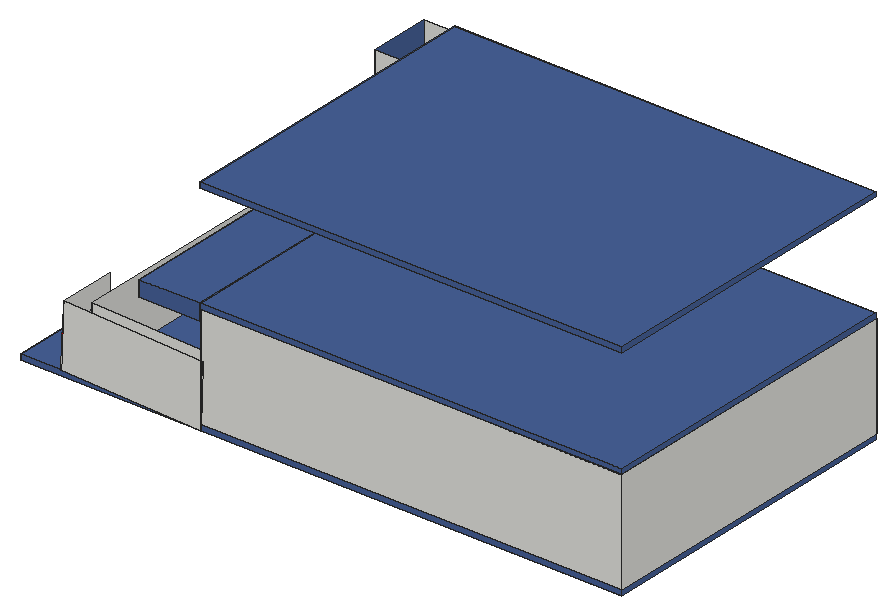
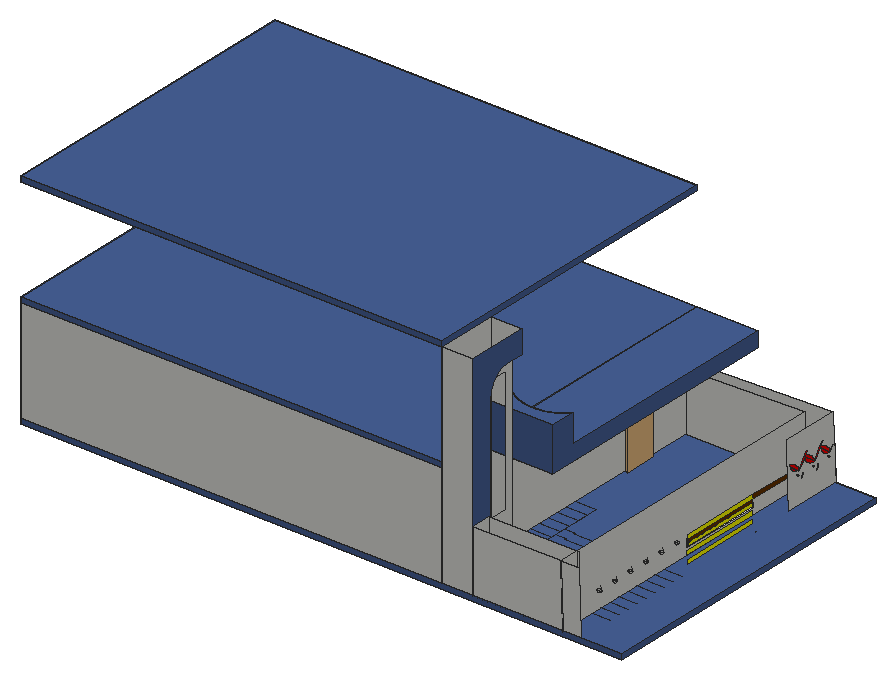
# SketchUp Ruby script. Lengths in inches.
U = 1.inch
M = Sketchup.active_model
def pt(a) = Geom::Point3d.new(a.map { |v| v * U })
def face(e, loops, mat)
  f = e.add_face(loops[0].map { |a| pt(a) })
  loops[1..].each { |l| e.add_face(l.map { |a| pt(a) }).erase! }
  f.material = f.back_material = mat if mat
  f
end
# faces: each face lists its corners as indices into pts; further lists are holes
def faces(e, pts, list, mat = nil) = list.each { |f| face(e, (f[0].is_a?(Array) ? f : [f]).map { |l| l.map { |i| pts[i] } }, mat) }
# xy, xz, yz: faces in a plane at the given z, y or x. An outline is a flat list of corners, or four numbers for a rectangle; further outlines are holes
def ring(l) = l.size == 4 ? [[l[0], l[1]], [l[2], l[1]], [l[2], l[3]], [l[0], l[3]]] : l.each_slice(2).to_a
def flat(e, list, mat, &to3) = list.each { |f| face(e, (f[0].is_a?(Array) ? f : [f]).map { |l| ring(l).map { |u, v| to3.(u, v) } }, mat) }
def xy(e, z, list, mat = nil) = flat(e, list, mat) { |x, y| [x, y, z] }
def xz(e, y, list, mat = nil) = flat(e, list, mat) { |x, z| [x, y, z] }
def yz(e, x, list, mat = nil) = flat(e, list, mat) { |y, z| [x, y, z] }
def lines(e, pts, list) = list.each { |a, b| e.add_line(pt(pts[a]), pt(pts[b])) }
# prism: a flat outline (further loops are holes) pulled along v
def prism(e, loops, v, mat = nil)
  f = face(e, loops, mat); d = Geom::Vector3d.new(v.map { |x| x * U })
  f.pushpull(f.normal.samedirection?(d) ? d.length : -d.length)
end
def box(e, o, s, mat = nil) = prism(e, [[o, [o[0] + s[0], o[1], o[2]], [o[0] + s[0], o[1] + s[1], o[2]], [o[0], o[1] + s[1], o[2]]]], [0, 0, s[2]], mat)
def at(x, y, z, deg = 0) = Geom::Transformation.translation(pt([x, y, z])) * Geom::Transformation.rotation(ORIGIN, Z_AXIS, deg.degrees)
def axes(o, x, y, z) = Geom::Transformation.new([*x, 0, *y, 0, *z, 0, *pt(o).to_a, 1])
def part(name) = M.definitions.add(name)
# library, detail: a bought-in or finely detailed component or shape, given as its bounding box
def library(name, o, s) = part(name).tap { |d| box(d.entities, o, s) }
def detail(e, o, s) = box(e.add_group.entities, o, s)
def put(e, d, t, mat = nil) = e.add_instance(d, t).tap { |i| i.material = mat if mat }
def group(e, t, mat = nil) = e.add_group.tap { |g| g.transformation = t; g.material = mat if mat }.entities
root = M.entities
M.materials.add("[Color A05]").color = [255, 0, 0]
M.materials.add("[Color C08]").color = [102, 51, 0]
M.materials.add("[Color E05]").color = [255, 255, 0]
M.materials.add("[Formica Blue]").color = [71, 97, 152]
xy(root,0,[[185,297.869,185,343.922,173,343.922,173,369.138,209,369.138,209,297.869],[47.3125,345.826,68.594,369.138],[68.656,345.826,173,369.138]])
xz(root,0.138,[[209,-6,211.689,66.45,50.001,72.45,48.995,45.334,48.867,41.896,48.729,38.166,48.499,31.965,48.496,31.88,48.384,28.884,47.3125,0]])
xz(root,15.244,[[209,-6,68.627,-0.791,71.315,71.659,211.689,66.45]])
xz(root,119.2,[[49.261,25.536,48.261,25.573,48.419,29.829,49.419,29.792]])
xz(root,213.237,[[49.261,25.536,49.419,29.792,48.419,29.829,48.261,25.573],[49.419,29.798,49.577,34.054,48.578,34.091,48.42,29.835]])
xz(root,297.869,[[185,0,209,0,209,246,173,246,173,219.281,185,219.281]])
xz(root,343.922,[[173,0,185,193.673]])
xz(root,345.826,[[68.656,0,173,71.758]])
xz(root,369.138,[[68.627,-0.791,47.3125,0,50.001,72.45,68.656,71.758,68.942,71.747,71.315,71.659,68.656,0],[68.656,0,71.315,71.659,68.942,71.747,69.797,71.758,173,71.758,173,0],[173,0,209,246]])
yz(root,173,[[345.826,0,369.138,71.758]])
yz(root,173,[[343.922,0,343.922,193.673,343.703,197.015,343.049,200.3,341.972,203.472,340.491,206.477,338.63,209.262,336.421,211.78,333.903,213.989,331.118,215.85,328.113,217.331,324.942,218.408,321.656,219.062,318.314,219.281,297.869,219.281,297.869,246,369.138,246,369.138,71.758,345.826,71.758,345.826,0]],"[Formica Blue]")
yz(root,185,[[[297.869,0,297.869,219.281,318.314,219.281,321.656,219.062,324.942,218.408,328.113,217.331,331.118,215.85,333.903,213.989,336.421,211.78,338.63,209.262,340.491,206.477,341.972,203.472,343.049,200.3,343.703,197.015,343.922,193.673,343.922,0],[306.65,57.692,336.962,201.38]]])
yz(root,209,[[297.869,0,369.138,246]])
p = [[68.627,15.244,-0.791],[209,15.244,-6],[209,0.138,-6],[47.3125,0.138,0],[47.3125,68.062,0],[47.3125,119.2,0],
  [48.312,119.2,-0.037],[48.312,213.237,-0.037],[47.3125,213.237,0],[47.3125,223.013,0],[47.3125,227.576,0],[47.3125,236.013,0],
  [47.3125,249.013,0],[47.3125,262.013,0],[47.3125,275.013,0],[47.3125,288.013,0],[47.3125,301.013,0],[47.3125,314.013,0],
  [47.3125,327.013,0],[47.3125,345.826,0],[47.3125,369.138,0],[68.627,369.138,-0.791],[211.689,15.244,66.45],[211.689,0.138,66.45],
  [68.656,369.138,0],[71.315,369.138,71.659],[71.315,15.244,71.659],[50.001,0.138,72.45],[50.001,68.062,72.45],[49.843,68.062,68.194],
  [49.843,68.062,68.188],[49.685,68.062,63.932],[49.685,68.062,63.926],[49.527,68.062,59.67],[49.527,68.062,59.664],[49.369,68.062,55.408],
  [49.368,68.062,55.402],[49.21,68.062,51.146],[49.21,68.062,51.139],[49.052,68.062,46.884],[49.052,68.062,46.877],[48.894,68.062,42.621],
  [48.894,68.062,42.615],[48.736,68.062,38.359],[48.736,68.062,38.353],[48.578,68.062,34.097],[48.578,68.062,34.091],[48.42,68.062,29.835],
  [48.419,68.062,29.829],[48.261,68.062,25.573],[48.261,68.062,25.567],[48.103,68.062,21.311],[48.103,68.062,21.304],[47.945,68.062,17.049],
  [47.945,68.062,17.042],[47.787,68.062,12.786],[47.787,68.062,12.78],[47.629,68.062,8.524],[47.629,68.062,8.518],[47.471,68.062,4.262],
  [47.47,68.062,4.256],[48.384,0.138,28.884],[48.496,0.138,31.88],[48.499,0.138,31.965],[48.729,0.138,38.166],[48.867,0.138,41.896],
  [48.995,0.138,45.334],[48.943,65.731,43.946],[49.003,66.251,45.543],[48.57,51.485,33.893],[48.575,53.16,34.028],[48.587,54.81,34.34],
  [48.605,56.418,34.827],[48.629,57.965,35.482],[48.659,59.432,36.299],[48.695,60.805,37.267],[48.737,62.066,38.376],[48.782,63.201,39.613],
  [48.833,64.198,40.965],[48.886,65.044,42.414],[48.954,20.801,44.237],[48.976,20.329,44.835],[48.928,18.683,43.536],[48.57,6.46,33.893],
  [48.575,8.135,34.028],[48.587,9.785,34.34],[48.605,11.393,34.827],[48.629,12.94,35.482],[48.659,14.407,36.299],[48.695,15.78,37.267],
  [48.737,17.041,38.376],[48.782,18.176,39.613],[48.833,19.173,40.965],[48.864,19.67,41.816],[48.886,20.019,42.414],[48.943,20.706,43.946],
  [48.928,41.195,43.536],[48.57,28.973,33.893],[48.575,30.647,34.028],[48.587,32.298,34.34],[48.605,33.906,34.827],[48.629,35.452,35.482],
  [48.659,36.92,36.299],[48.695,38.292,37.267],[48.737,39.553,38.376],[48.782,40.688,39.613],[48.833,41.685,40.965],[48.864,42.182,41.816],
  [48.908,41.459,43.009],[48.632,28.559,35.558],[48.692,28.017,37.186],[48.751,27.352,38.767],[48.808,26.567,40.292],[48.862,25.666,41.753],
  [48.913,24.655,43.139],[48.962,23.54,44.443],[49.007,22.328,45.658],[49.048,21.025,46.775],[49.086,19.64,47.789],[49.119,18.182,48.693],
  [49.149,16.657,49.482],[49.003,21.226,45.543],[48.343,28.077,27.775],[48.116,27.182,21.657],[48.153,27.246,22.641],[48.189,27.225,23.627],
  [48.226,27.119,24.607],[48.262,26.927,25.574],[48.297,26.652,26.521],[48.331,26.296,27.44],[48.364,25.861,28.325],[48.395,25.351,29.169],
  [48.424,24.77,29.966],[48.452,24.121,30.709],[48.477,23.41,31.392],[48.5,22.643,32.012],[48.464,22.5625,31.026],[48.427,22.571,30.037],
  [48.391,22.668,29.053],[48.355,22.853,28.082],[48.319,23.125,27.131],[48.285,23.481,26.208],[48.252,23.918,25.321],[48.221,24.434,24.477],
  [48.191,25.023,23.682],[48.164,25.681,22.943],[48.139,26.402,22.266],[48.34,50.518,27.681],[48.113,49.622,21.563],[48.149,49.687,22.547],
  [48.186,49.666,23.532],[48.222,49.559,24.512],[48.258,49.368,25.48],[48.293,49.093,26.426],[48.327,48.736,27.346],[48.36,48.302,28.231],
  [48.391,47.792,29.075],[48.421,47.21,29.871],[48.449,46.562,30.614],[48.474,45.851,31.298],[48.497,45.083,31.918],[48.46,45.003,30.932],
  [48.424,45.012,29.943],[48.387,45.109,28.959],[48.351,45.294,27.987],[48.316,45.566,27.036],[48.282,45.922,26.114],[48.249,46.359,25.227],
  [48.217,46.874,24.382],[48.188,47.463,23.588],[48.16,48.121,22.849],[48.135,48.843,22.172],[48.854,42.353,41.535],[48.802,43.365,40.14],
  [48.753,44.489,38.832],[48.709,45.716,37.62],[48.667,47.038,36.514],[48.631,48.447,35.52],[48.598,49.933,34.644],[48.954,43.313,44.237],
  [48.943,43.219,43.946],[48.886,42.532,42.414],[48.368,28.237,28.44],[48.345,28.728,27.816],[48.349,29.371,27.92],[48.355,30.001,28.087],
  [48.363,30.611,28.316],[48.374,31.196,28.603],[48.387,31.75,28.947],[48.401,32.267,29.344],[48.418,32.742,29.789],[48.436,33.172,30.279],
  [48.456,33.55,30.809],[48.477,33.875,31.374],[48.499,34.142,31.968],[48.502,33.464,32.053],[48.502,32.779,32.048],[48.498,32.102,31.952],
  [48.491,31.443,31.767],[48.481,30.815,31.497],[48.468,30.228,31.146],[48.453,29.692,30.721],[48.434,29.217,30.228],[48.414,28.812,29.677],
  [48.392,28.484,29.078],[48.364,50.678,28.346],[48.341,51.168,27.721],[48.345,51.812,27.826],[48.351,52.442,27.993],[48.36,53.052,28.222],
  [48.37,53.637,28.509],[48.383,54.191,28.853],[48.398,54.708,29.249],[48.414,55.183,29.695],[48.433,55.612,30.185],[48.452,55.991,30.715],
  [48.473,56.316,31.28],[48.495,56.583,31.874],[48.498,55.904,31.959],[48.498,55.22,31.953],[48.495,54.543,31.857],[48.488,53.884,31.673],
  [48.478,53.255,31.403],[48.465,52.668,31.052],[48.449,52.133,30.626],[48.431,51.658,30.134],[48.41,51.253,29.583],[48.388,50.924,28.983],
  [48.368,5.675,28.44],[48.343,5.515,27.775],[48.345,6.165,27.816],[48.349,6.809,27.92],[48.355,7.439,28.087],[48.363,8.049,28.316],
  [48.374,8.634,28.603],[48.387,9.1875,28.947],[48.401,9.704,29.344],[48.418,10.18,29.789],[48.436,10.609,30.279],[48.456,10.988,30.809],
  [48.477,11.3125,31.374],[48.499,11.58,31.968],[48.502,10.901,32.053],[48.502,10.217,32.048],[48.498,9.54,31.952],[48.491,8.881,31.767],
  [48.481,8.252,31.497],[48.468,7.665,31.146],[48.453,7.13,30.721],[48.434,6.655,30.228],[48.414,6.25,29.677],[48.392,5.921,29.078],
  [48.976,42.841,44.835],[49.149,39.17,49.482],[49.086,39.54,47.799],[49.025,40.048,46.151],[48.966,40.689,44.551],[49.003,43.738,45.543],
  [48.786,213.237,12.743],[48.628,213.237,8.487],[48.628,119.2,8.487],[48.786,119.2,12.743],[49.102,213.237,21.267],[48.944,213.237,17.011],
  [48.944,119.2,17.011],[49.102,119.2,21.267],[48.261,213.237,25.573],[48.261,119.2,25.573],[49.261,119.2,25.536],[49.261,213.237,25.536],
  [49.419,213.237,29.792],[49.419,119.2,29.792],[48.419,119.2,29.829],[48.419,213.237,29.829],[48.42,213.237,29.835],[48.42,119.2,29.835],
  [49.419,119.2,29.798],[49.419,213.237,29.798],[49.577,213.237,34.054],[49.577,119.2,34.054],[48.709,0.691,37.62],[48.598,4.908,34.644],
  [48.631,3.422,35.52],[48.667,2.013,36.514],[48.962,1.027,44.443],[48.913,2.142,43.139],[48.862,3.153,41.753],[48.808,4.054,40.292],
  [48.751,4.84,38.767],[48.692,5.505,37.186],[48.632,6.046,35.558],[48.908,18.946,43.009],[48.587,7.025,35.463],[48.608,7.746,36.967],
  [48.633,8.615,38.39],[48.663,9.624,39.718],[48.696,10.761,40.9375],[48.733,12.016,42.035],[48.773,13.376,43],[48.815,14.827,43.823],
  [48.86,16.353,44.495],[48.906,17.939,45.008],[48.954,19.569,45.359],[48.854,19.841,41.535],[48.598,27.42,34.644],[48.631,25.935,35.52],
  [48.667,24.526,36.514],[48.709,23.203,37.62],[48.753,21.976,38.832],[48.802,20.853,40.14],[48.587,29.538,35.463],[48.608,30.259,36.967],
  [48.633,31.128,38.39],[48.663,32.136,39.718],[48.696,33.274,40.9375],[48.733,34.529,42.035],[48.773,35.889,43],[48.815,37.339,43.823],
  [48.86,38.865,44.495],[48.906,40.451,45.008],[48.954,42.081,45.359],[49.119,40.694,48.693],[49.086,42.153,47.789],[49.048,43.538,46.775],
  [49.007,44.84,45.658],[48.962,46.052,44.443],[48.913,47.167,43.139],[48.862,48.178,41.753],[48.808,49.079,40.292],[48.751,49.865,38.767],
  [48.692,50.53,37.186],[48.632,51.071,35.558],[48.587,52.05,35.463],[48.608,52.771,36.967],[48.633,53.64,38.39],[48.663,54.649,39.718],
  [48.696,55.786,40.9375],[48.733,57.041,42.035],[48.773,58.401,43],[48.815,59.852,43.823],[48.86,61.378,44.495],[48.906,62.964,45.008],
  [48.954,64.594,45.359],[48.736,119.2,38.353],[48.578,119.2,34.097],[48.736,213.237,38.353],[48.578,213.237,34.097],[48.578,119.2,34.091],
  [48.578,213.237,34.091],[48.585,338.004,34.285],[48.74,344.07,38.478],[48.718,343.802,37.884],[48.697,343.478,37.319],[48.678,343.099,36.789],
  [48.66,342.67,36.299],[48.643,342.194,35.853],[48.628,341.677,35.457],[48.616,341.123,35.113],[48.605,340.539,34.826],[48.596,339.928,34.597],
  [48.59,339.298,34.43],[48.586,338.655,34.325],[48.609,338.164,34.95],[48.633,338.411,35.587],[48.655,338.739,36.187],[48.676,339.145,36.738],
  [48.694,339.619,37.23],[48.71,340.155,37.656],[48.723,340.742,38.007],[48.733,341.37,38.277],[48.74,342.029,38.461],[48.743,342.707,38.557],
  [48.744,343.391,38.563],[48.588,225.514,34.379],[48.744,231.579,38.572],[48.722,231.312,37.978],[48.701,230.987,37.413],[48.681,230.608,36.883],
  [48.663,230.179,36.393],[48.646,229.704,35.948],[48.632,229.186,35.551],[48.619,228.633,35.207],[48.608,228.048,34.92],[48.6,227.4375,34.691],
  [48.594,226.808,34.524],[48.59,226.164,34.42],[48.613,225.674,35.044],[48.637,225.92,35.682],[48.659,226.249,36.281],[48.679,226.654,36.832],
  [48.698,227.129,37.325],[48.713,227.664,37.75],[48.726,228.251,38.101],[48.736,228.88,38.371],[48.743,229.539,38.556],[48.747,230.216,38.652],
  [48.747,230.9,38.657],[48.588,248.026,34.379],[48.744,254.091,38.572],[48.722,253.824,37.978],[48.701,253.499,37.413],[48.681,253.121,36.883],
  [48.663,252.691,36.393],[48.646,252.216,35.948],[48.632,251.699,35.551],[48.619,251.145,35.207],[48.608,250.56,34.92],[48.6,249.95,34.691],
  [48.594,249.32,34.524],[48.59,248.677,34.42],[48.613,248.186,35.044],[48.637,248.433,35.682],[48.659,248.761,36.281],[48.679,249.167,36.832],
  [48.698,249.641,37.325],[48.713,250.177,37.75],[48.726,250.764,38.101],[48.736,251.392,38.371],[48.743,252.051,38.556],[48.747,252.729,38.652],
  [48.747,253.413,38.657],[48.588,270.489,34.379],[48.744,276.554,38.572],[48.722,276.287,37.978],[48.701,275.962,37.413],[48.681,275.583,36.883],
  [48.663,275.154,36.393],[48.646,274.679,35.948],[48.632,274.161,35.551],[48.619,273.608,35.207],[48.608,273.023,34.92],[48.6,272.413,34.691],
  [48.594,271.783,34.524],[48.59,271.139,34.42],[48.613,270.649,35.044],[48.637,270.895,35.682],[48.659,271.224,36.281],[48.679,271.629,36.832],
  [48.698,272.104,37.325],[48.713,272.639,37.75],[48.726,273.226,38.101],[48.736,273.855,38.371],[48.743,274.514,38.556],[48.747,275.191,38.652],
  [48.747,275.875,38.657],[48.588,293.001,34.379],[48.744,299.066,38.572],[48.722,298.799,37.978],[48.701,298.474,37.413],[48.681,298.096,36.883],
  [48.663,297.666,36.393],[48.646,297.191,35.948],[48.632,296.674,35.551],[48.619,296.12,35.207],[48.608,295.535,34.92],[48.6,294.925,34.691],
  [48.594,294.295,34.524],[48.59,293.652,34.42],[48.613,293.161,35.044],[48.637,293.408,35.682],[48.659,293.736,36.281],[48.679,294.142,36.832],
  [48.698,294.616,37.325],[48.713,295.152,37.75],[48.726,295.739,38.101],[48.736,296.367,38.371],[48.743,297.026,38.556],[48.747,297.704,38.652],
  [48.747,298.388,38.657],[48.588,315.564,34.379],[48.744,321.629,38.572],[48.722,321.362,37.978],[48.701,321.037,37.413],[48.681,320.658,36.883],
  [48.663,320.229,36.393],[48.646,319.754,35.948],[48.632,319.236,35.551],[48.619,318.683,35.207],[48.608,318.098,34.92],[48.6,317.488,34.691],
  [48.594,316.858,34.524],[48.59,316.214,34.42],[48.613,315.724,35.044],[48.637,315.97,35.682],[48.659,316.299,36.281],[48.679,316.704,36.832],
  [48.698,317.179,37.325],[48.713,317.714,37.75],[48.726,318.301,38.101],[48.736,318.93,38.371],[48.743,319.589,38.556],[48.747,320.266,38.652],
  [48.747,320.95,38.657],[68.594,345.826,0],[68.656,345.826,0],[48.812,338.9,40.403],[48.815,316.46,40.497],[48.815,293.897,40.497],
  [48.815,271.385,40.497],[48.815,248.922,40.497],[68.594,327.013,0],[68.656,327.013,0],[173,327.013,0],[209,279.056,0],
  [185,279.056,0],[173,325.109,0],[185,325.109,0],[68.656,314.013,0],[173,314.013,0],[68.594,314.013,0],
  [209,266.056,0],[185,266.056,0],[173,312.109,0],[185,312.109,0],[68.656,301.013,0],[173,301.013,0],
  [68.594,301.013,0],[209,253.056,0],[185,253.056,0],[173,299.109,0],[185,299.109,0],[68.656,288.013,0],
  [173,288.013,0],[68.594,288.013,0],[209,240.056,0],[185,240.056,0],[173,286.109,0],[185,286.109,0],
  [185,297.869,0],[185,284.869,0],[68.656,275.013,0],[173,275.013,0],[68.594,275.013,0],[209,227.056,0],
  [185,227.056,0],[173,273.109,0],[185,273.109,0],[185,271.869,0],[68.656,262.013,0],[173,262.013,0],
  [68.594,262.013,0],[209,214.056,0],[185,214.056,0],[173,260.109,0],[185,260.109,0],[185,258.869,0],
  [68.656,249.013,0],[173,249.013,0],[68.594,249.013,0],[209,201.056,0],[185,201.056,0],[173,247.109,0],
  [185,247.109,0],[185,245.869,0],[68.656,236.013,0],[173,236.013,0],[68.594,236.013,0],[209,188.056,0],
  [185,188.056,0],[173,234.109,0],[185,234.109,0],[185,232.869,0],[68.656,223.013,0],[173,223.013,0],
  [68.594,223.013,0],[185,193.869,0],[185,175.056,0],[209,175.056,0],[173,221.109,0],[185,221.109,0],
  [185,206.869,0],[185,219.869,0],[208.755,10.382,-6.604],[208.755,81.651,-6.604]]
faces(root,p,[[0,1,2,3,4,5,6,7,8,9,10,11,12,13,14,15,16,17,18,19,20,21],[2,1,22,23],[0,21,24,25,26],[[27,28,29,30,31,32,33,34,35,36,37,38,39,40,41,42,43,44,45,46,47,48,49,50,51,52,53,54,55,56,57,58,59,60,4,3,61,62,63,64,65,66],[67,68,69,70,71,72,73,74,75,76,77,78,79],[80,81,82,83,84,85,86,87,88,89,90,91,92,93,94,95],[96,97,98,99,100,101,102,103,104,105,106,107,108],[80,97,109,110,111,112,113,114,115,116,117,118,119,120,81,121],[122,123,124,125,126,127,128,129,130,131,132,133,134,135,136,137,138,139,140,141,142,143,144,145,146,123],[147,148,149,150,151,152,153,154,155,156,157,158,159,160,161,162,163,164,165,166,167,168,169,170,171,148],[107,172,173,174,175,176,177,178,69,179,180,181],[182,122,183,184,185,186,187,188,189,190,191,192,193,194,195,196,197,198,199,200,201,202,203,204],[205,147,206,207,208,209,210,211,212,213,214,215,216,217,218,219,220,221,222,223,224,225,226,227],[228,229,230,231,232,233,234,235,236,237,238,239,240,241,242,243,244,245,246,247,248,249,250,251],[252,253,254,255,256,96],[252,179,257]],[266,267,268,269],[272,273,270,271],[274,275,276,277],[347,348,278,279],
  [349,350,351,352,353,354,355,356,357,358,359,360,361],[350,349,362,363,364,365,366,367,368,369,370,371,372],[373,374,375,376,377,378,379,380,381,382,383,384,385],[374,373,386,387,388,389,390,391,392,393,394,395,396],[397,398,399,400,401,402,403,404,405,406,407,408,409],[398,397,410,411,412,413,414,415,416,417,418,419,420],[421,422,423,424,425,426,427,428,429,430,431,432,433],[422,421,434,435,436,437,438,439,440,441,442,443,444],
  [445,446,447,448,449,450,451,452,453,454,455,456,457],[446,445,458,459,460,461,462,463,464,465,466,467,468],[469,470,471,472,473,474,475,476,477,478,479,480,481],[470,469,482,483,484,485,486,487,488,489,490,491,492]])
faces(root,p,[[258,259,260,261],[262,263,264,265],[270,269,268,271],[345,346,344,343]],"[Color E05]")
faces(root,p,[[278,277,276,279],[343,344,45,44]],"[Color C08]")
faces(root,p,[[280,64,65,83,281,282,283],[83,65,66,284,285,286,287,288,289,290],[83,82,291,93,92,91,90,89,88,87,86,85,84],[82,83,292,293,294,295,296,297,298,299,300,301,302,121,81],[97,80,121,81,120,119,118,117,116,115,114,113,112,111,110,109],[303,93,94,95,80,97,304,305,306,307,308,309],[97,96,108,107,106,105,104,103,102,101,100,99,98],[96,97,310,311,312,313,314,315,316,317,318,319,320,257,252],
  [69,179,257,252,253,321,322,323,324,325,326,327,328,329,330,331],[172,107,181,180,179,69,178,177,176,175,174,173],[68,67,79,78,77,76,75,74,73,72,71,70,69],[68,69,332,333,334,335,336,337,338,339,340,341,342]],"[Color A05]")
lines(root,p,[[493,494],[495,349],[496,469],[497,445],[498,421],[499,397],[500,501],[18,500],[501,502],[503,504],[505,502],[506,505],
  [507,508],[17,509],[509,507],[510,511],[512,508],[513,512],[514,515],[16,516],[516,514],[517,518],[519,515],[520,519],
  [521,522],[15,523],[523,521],[524,525],[526,522],[527,526],[527,528],[504,529],[529,527],[530,531],[14,532],[532,530],
  [533,534],[535,531],[536,535],[536,504],[511,537],[537,536],[538,539],[13,540],[540,538],[541,542],[543,539],[544,543],
  [544,511],[518,545],[545,544],[546,547],[12,548],[548,546],[549,550],[551,547],[552,551],[552,518],[525,553],[553,552],
  [554,555],[11,556],[556,554],[557,558],[559,555],[560,559],[560,525],[534,561],[561,560],[562,563],[9,564],[564,562],
  [565,550],[566,558],[567,566],[568,563],[569,568],[569,534],[550,570],[558,565],[570,542],[542,571],[571,569],[572,573]])
detail(root,[205.5,67.97,0],[3.5,36,84])
g1 = group(root,at(85.08,-1102.71,0),"[Formica Blue]")
xy(g1,107.8125,[[52.54,1102.85,123.48,1400.58]])
xy(g1,126,[[52.54,1102.85,123.48,1371.64],[52.54,1371.64,123.48,1371.64,118.54,1375.95,113.08,1379.58,107.2,1382.46,100.99,1384.5625,94.55,1385.84,88.01,1386.26,81.47,1385.84,75.04,1384.5625,68.83,1382.46,62.95,1379.58,57.49,1375.95]])
xy(g1,158.1875,[[52.54,1371.64,57.49,1375.95,62.95,1379.58,68.83,1382.46,75.04,1384.5625,81.47,1385.84,88.01,1386.26,94.55,1385.84,100.99,1384.5625,107.2,1382.46,113.08,1379.58,118.54,1375.95,123.48,1371.64,123.48,1400.58,52.54,1400.58]])
xz(g1,1102.85,[[52.54,107.8125,123.48,126]])
xz(g1,1400.58,[[52.54,107.8125,123.48,158.1875]])
yz(g1,52.54,[[1102.85,107.8125,1102.85,126,1371.64,126,1371.64,158.1875,1400.58,158.1875,1400.58,107.8125]])
yz(g1,123.48,[[1102.85,107.8125,1400.58,107.8125,1400.58,158.1875,1371.64,158.1875,1371.64,126,1102.85,126]])
p = [[57.49,1375.95,158.1875],[52.54,1371.64,158.1875],[52.54,1371.64,126],[57.49,1375.95,126],[123.48,1371.64,158.1875],[118.54,1375.95,158.1875],
  [118.54,1375.95,126],[123.48,1371.64,126],[62.95,1379.58,158.1875],[62.95,1379.58,126],[113.08,1379.58,158.1875],[113.08,1379.58,126],
  [68.83,1382.46,158.1875],[68.83,1382.46,126],[107.2,1382.46,158.1875],[107.2,1382.46,126],[75.04,1384.5625,158.1875],[75.04,1384.5625,126],
  [100.99,1384.5625,158.1875],[100.99,1384.5625,126],[81.47,1385.84,158.1875],[81.47,1385.84,126],[94.55,1385.84,158.1875],[94.55,1385.84,126],
  [88.01,1386.26,158.1875],[88.01,1386.26,126]]
faces(g1,p,[[0,1,2,3],[4,5,6,7],[8,0,3,9],[5,10,11,6],[12,8,9,13],[10,14,15,11],[16,12,13,17],[14,18,19,15],
  [20,16,17,21],[18,22,23,19],[24,20,21,25],[22,24,25,23]])
g2 = group(g1,at(123.92,1102.85,-6))
box(g2,[-209,0,0],[698,369,6])
g3 = group(g1,at(123.48,1102.85,120))
box(g3,[0,0,0],[489,369,6])
g4 = group(g1,at(123.48,1102.85,246))
box(g4,[0,0,0],[489,369,6])
g5 = group(root,at(209,0.14,0))
xy(g5,0,[[0,0,489,0,489,369,0,369,0,150.65,9,150.65,9,360,480,360,480,9,9,9,9,67.83,0,67.83],[9,9,480,360],[0,67.83,9,103.83]])
xy(g5,42,[[0,150.65,9,210.65]])
xy(g5,84,[[0,67.83,9,103.83],[0,150.65,9,210.65]])
xy(g5,120,[[0,0,489,0,489,369,0,369,0,67.83,9,67.83,9,360,480,360,480,9,9,9,9,67.83,0,67.83]])
xz(g5,0,[[0,0,489,120]])
xz(g5,9,[[9,0,480,120]])
xz(g5,67.83,[[0,0,9,84]])
xz(g5,103.83,[[0,0,9,84]])
xz(g5,150.65,[[0,42,9,84]])
xz(g5,210.65,[[0,42,9,84]])
xz(g5,360,[[9,0,480,120]])
xz(g5,369,[[0,0,489,120]])
yz(g5,0,[[[0,0,0,120,369,120,369,0,103.83,0,103.83,84,67.83,84,67.83,0],[150.65,42,210.65,84]]])
yz(g5,9,[[9,0,67.83,120],[[103.83,0,360,0,360,120,67.83,120,67.83,84,103.83,84],[150.65,42,210.65,84]]])
yz(g5,480,[[9,0,360,120]])
yz(g5,489,[[0,0,369,120]])
